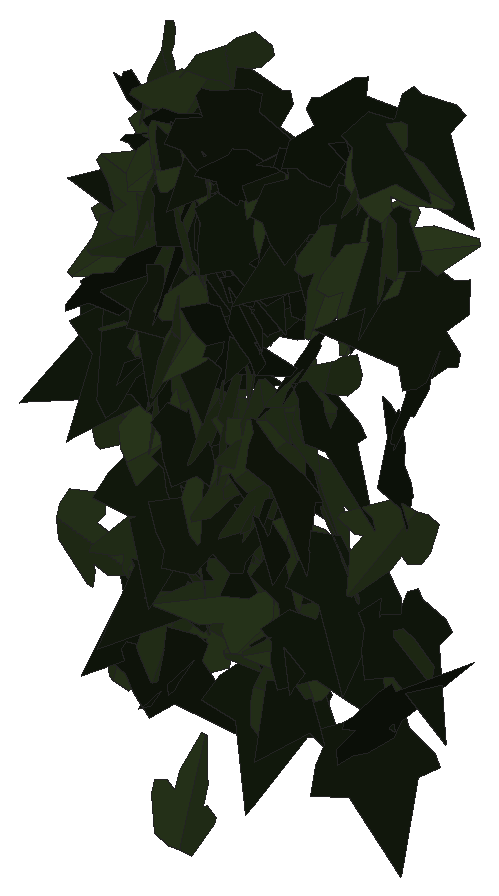
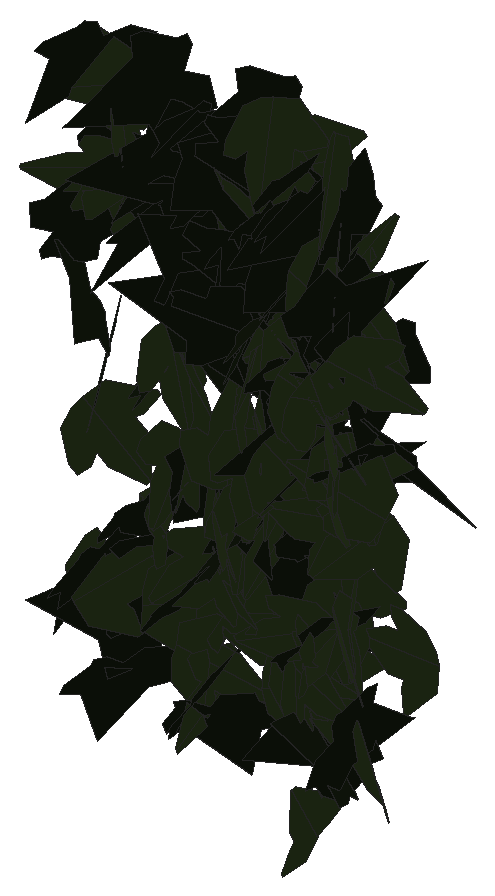
# SketchUp Ruby script. Lengths in inches.
U = 1.inch
M = Sketchup.active_model
def pt(a) = Geom::Point3d.new(a.map { |v| v * U })
def face(e, loops, mat)
  f = e.add_face(loops[0].map { |a| pt(a) })
  loops[1..].each { |l| e.add_face(l.map { |a| pt(a) }).erase! }
  f.material = f.back_material = mat if mat
  f
end
# faces: each face lists its corners as indices into pts; further lists are holes
def faces(e, pts, list, mat = nil) = list.each { |f| face(e, (f[0].is_a?(Array) ? f : [f]).map { |l| l.map { |i| pts[i] } }, mat) }
# xy, xz, yz: faces in a plane at the given z, y or x. An outline is a flat list of corners, or four numbers for a rectangle; further outlines are holes
def ring(l) = l.size == 4 ? [[l[0], l[1]], [l[2], l[1]], [l[2], l[3]], [l[0], l[3]]] : l.each_slice(2).to_a
def flat(e, list, mat, &to3) = list.each { |f| face(e, (f[0].is_a?(Array) ? f : [f]).map { |l| ring(l).map { |u, v| to3.(u, v) } }, mat) }
def xy(e, z, list, mat = nil) = flat(e, list, mat) { |x, y| [x, y, z] }
def xz(e, y, list, mat = nil) = flat(e, list, mat) { |x, z| [x, y, z] }
def yz(e, x, list, mat = nil) = flat(e, list, mat) { |y, z| [x, y, z] }
def lines(e, pts, list) = list.each { |a, b| e.add_line(pt(pts[a]), pt(pts[b])) }
# prism: a flat outline (further loops are holes) pulled along v
def prism(e, loops, v, mat = nil)
  f = face(e, loops, mat); d = Geom::Vector3d.new(v.map { |x| x * U })
  f.pushpull(f.normal.samedirection?(d) ? d.length : -d.length)
end
def box(e, o, s, mat = nil) = prism(e, [[o, [o[0] + s[0], o[1], o[2]], [o[0] + s[0], o[1] + s[1], o[2]], [o[0], o[1] + s[1], o[2]]]], [0, 0, s[2]], mat)
def at(x, y, z, deg = 0) = Geom::Transformation.translation(pt([x, y, z])) * Geom::Transformation.rotation(ORIGIN, Z_AXIS, deg.degrees)
def axes(o, x, y, z) = Geom::Transformation.new([*x, 0, *y, 0, *z, 0, *pt(o).to_a, 1])
def part(name) = M.definitions.add(name)
# library, detail: a bought-in or finely detailed component or shape, given as its bounding box
def library(name, o, s) = part(name).tap { |d| box(d.entities, o, s) }
def detail(e, o, s) = box(e.add_group.entities, o, s)
def put(e, d, t, mat = nil) = e.add_instance(d, t).tap { |i| i.material = mat if mat }
def group(e, t, mat = nil) = e.add_group.tap { |g| g.transformation = t; g.material = mat if mat }.entities
root = M.entities
M.materials.add("efeu1").color = [18, 25, 13]
M.materials.add("efeu2").color = [43, 57, 29]
c1 = part("ivyleaf_9")
p = [[1.54,2.16,1.25],[1.36,2.04,1.19],[-0.21,0.99,0.68],[-0.71,1.11,0.82],[-0.85,0.86,0.67],[-0.8,0.17,0.21],
  [-0.9,-0.01,0.1],[-0.67,-0.16,-0.02],[-0.08,-0.08,-0.05],[-0.03,-0.6,-0.4],[0.65,-0.88,-0.66],[0.83,-0.6,-0.49],
  [1.29,-0.42,-0.43],[1.8125,-0.07,-0.26],[1.21,0.44,0.15]]
faces(c1.entities,p,[[0,1,2,3,4,5,6,7,8,9,10,11,12,13,14]],"efeu1")
c2 = part("ivyleaf_10")
p = [[0,0.5,-0.03],[-0.0625,2.02,-0.43],[-0.19,2.01,-0.46],[-0.54,1.05,-0.29],[-0.52,0.625,-0.18],[-0.83,0.76,-0.28],
  [-1.16,0.64,-0.33],[-1.15,0.33,-0.24],[-0.77,-0.39,0.02],[-0.3,-0.51,0.16],[0.04,-0.48,0.23],[-0.02,2.01,-0.4375],
  [-0.06,2.01,-0.43],[0.04,-0.49,0.23],[0.67,-0.49,0.14],[1.38,0.36,-0.2],[1.375,0.51,-0.24],[0.81,0.65,-0.19],
  [0.62,0.59,-0.15],[0.6,1.09,-0.28],[0.5,1.23,-0.31]]
faces(c2.entities,p,[[0,1,2,3,4,5,6,7,8,9,10],[11,12,0,13,14,15,16,17,18,19,20]],"efeu2")
put(root,c1,axes([26,222.56,219.11],[-0.4769,0.10257,0.10975],[-0.10783,0.0206,-0.4878],[-0.10459,-0.48893,0.00247]))
put(root,c1,axes([27.44,222.25,222.61],[0.04677,0.071,-0.49272],[0.25531,0.42142,0.08496],[0.42735,-0.25954,0.00317]))
put(root,c2,axes([26.96,222.25,219.75],[0.05277,-0.33846,-0.36422],[-0.01811,0.36472,-0.34154],[0.49688,0.04924,0.02623]))
put(root,c1,axes([26.62,222.67,217.6875],[-0.32572,-0.33531,-0.17742],[0.13158,0.11946,-0.46735],[0.3558,-0.35114,0.01042]))
put(root,c2,axes([27.1,222.21,213.6875],[0.02192,0.38608,-0.31696],[0.03124,0.31558,0.38657],[0.49854,-0.03675,-0.01029]))
put(root,c1,axes([26.18,222.25,220.25],[0.13268,0.48116,-0.02974],[-0.0089,-0.02839,-0.49911],[-0.48199,0.13298,0.00103]))
put(root,c2,axes([29.8,222.7,218.16],[-0.20695,-0.34897,0.29222],[-0.12821,-0.26331,-0.40525],[0.43673,-0.24267,0.01951]))
put(root,c1,axes([29.0625,222.75,217.375],[-0.04611,-0.49762,0.01589],[0.00134,-0.01609,-0.49974],[0.49787,-0.04604,0.00282]))
put(root,c2,axes([28.99,222.66,221.34],[0.18709,0.39205,-0.24758],[-0.08922,-0.23154,-0.43408],[-0.45501,0.20661,-0.01668]))
put(root,c2,axes([26.875,222.55,222],[0.38106,-0.00662,-0.32365],[-0.32328,0.01813,-0.381],[0.01678,0.49963,0.00953]))
put(root,c1,axes([27.43,222.35,217.21],[-0.46658,0.06612,0.16711],[0.16511,-0.02591,0.47124],[0.07098,0.49493,0.00234]))
put(root,c2,axes([25.32,222.61,216.62],[-0.07292,0.04696,-0.49242],[0.44472,-0.2117,-0.08605],[-0.21657,-0.45053,-0.0109]))
put(root,c2,axes([26.47,222.54,217.01],[-0.29156,-0.40555,0.02281],[-0.0134,-0.01846,-0.49948],[0.40597,-0.29187,-0.00011]))
put(root,c2,axes([26.36,222.53,220.75],[-0.27482,-0.05765,0.4137],[-0.40528,-0.08308,-0.2808],[0.10112,-0.48967,-0.00107]))
put(root,c2,axes([27.125,222.7,219.99],[0.26993,0.30188,-0.29327],[-0.18987,-0.22359,-0.40492],[-0.37562,0.32996,-0.00608]))
put(root,c1,axes([28.76,222.65,219.31],[0.2713,-0.41997,0.00461],[0.0025,-0.00387,-0.49998],[0.41999,0.27131,0]))
put(root,c2,axes([27.6,222.75,216.51],[0.03345,0.0607,-0.49517],[-0.44165,-0.22719,-0.05768],[-0.232,0.44125,0.03841]))
put(root,c2,axes([26.92,222.71,222.54],[-0.23985,-0.37338,0.23035],[-0.09067,-0.21468,-0.44237],[0.42925,-0.25398,0.03527]))
put(root,c2,axes([29.45,222.63,221.3],[0.31072,0.35782,-0.15943],[-0.10236,-0.12227,-0.47389],[-0.37812,0.32714,-0.00273]))
put(root,c1,axes([26.65,222.93,216.49],[-0.2778,-0.34146,0.23713],[-0.12438,-0.20387,-0.43928],[0.39668,-0.30305,0.02833]))
put(root,c1,axes([27.11,222.59,216.83],[-0.15132,0.06294,0.47238],[0.38889,-0.27015,0.16057],[0.27544,0.416,0.03281]))
put(root,c2,axes([26.68,222.66,216.0625],[-0.23025,-0.42995,0.11013],[-0.04507,-0.10078,-0.48766],[0.44154,-0.23449,0.00765]))
put(root,c2,axes([28.72,222.86,216.29],[0.01115,0.03174,-0.49887],[-0.3673,-0.33794,-0.02971],[-0.33906,0.36713,0.01578]))
put(root,c2,axes([26.32,222.76,221],[-0.01761,0.38951,0.313],[-0.01688,-0.31348,0.38916],[0.4994,0.00314,0.02419]))
put(root,c2,axes([29.5,222.67,221.69],[0.43821,-0.2295,0.07282],[0.06865,-0.02585,-0.49459],[0.23078,0.44347,0.00885]))
put(root,c2,axes([27.96,222.73,218.4375],[-0.27935,-0.2078,0.35886],[-0.28085,-0.22354,-0.34807],[0.3051,-0.39604,0.00816]))
put(root,c1,axes([28.07,222.83,218.39],[0.14621,-0.46138,0.1255],[0.04153,-0.11848,-0.48398],[0.47634,0.15195,0.00368]))
put(root,c2,axes([26.51,222.4375,221.4375],[0.1581,-0.38696,-0.27435],[-0.02032,0.2834,-0.41143],[0.47391,0.14124,0.07388]))
put(root,c2,axes([26.97,222.74,221.39],[-0.26885,0.32414,-0.26954],[0.09475,-0.26505,-0.41324],[-0.41078,-0.27328,0.08109]))
put(root,c2,axes([26.95,222.45,221.16],[-0.23786,0.42093,0.12743],[-0.07019,0.10669,-0.48342],[-0.43416,-0.24786,0.00834]))
put(root,c1,axes([29.39,222.76,221.79],[-0.39357,-0.18904,-0.24365],[0.21736,0.11019,-0.43659],[0.21877,-0.44958,-0.00455]))
put(root,c2,axes([27.35,222.8125,218.93],[0.24503,-0.3728,0.22579],[0.15753,-0.16577,-0.44464],[0.40638,0.28904,0.03622]))
put(root,c1,axes([28.76,222.95,221.39],[-0.40449,-0.22677,0.18698],[-0.14051,-0.13019,-0.46185],[0.25816,-0.42617,0.04159]))
put(root,c1,axes([27,222.53,219.64],[0.19931,0.13211,-0.43911],[0.35027,0.26515,0.23876],[0.29595,-0.40279,0.01314]))
put(root,c1,axes([28.77,222.53,216.64],[-0.11176,-0.1846,-0.45104],[0.19886,0.40519,-0.21511],[0.44493,-0.22747,-0.01715]))
put(root,c1,axes([27.5625,222.65,221.32],[0.12738,-0.42197,-0.23605],[-0.07208,0.2248,-0.44076],[0.4781,0.14632,-0.00355]))
put(root,c1,axes([26.03,223,218.98],[-0.31516,-0.35453,0.15808],[-0.05816,-0.15819,-0.47074],[0.38379,-0.3151,0.05847]))
put(root,c1,axes([26.12,222.86,221.87],[0.11032,-0.18095,0.45287],[0.30189,-0.33931,-0.20912],[0.38301,0.31957,0.03439]))
put(root,c1,axes([29.53,223.04,218.68],[0.00274,-0.12171,0.48495],[0.00376,-0.48494,-0.12173],[0.49998,0.00431,-0.00174]))
put(root,c1,axes([27.5,222.7,220.27],[0.02691,0.08722,-0.4916],[-0.41095,-0.27572,-0.07142],[-0.28355,0.40788,0.05685]))
put(root,c1,axes([26.8,222.86,219.98],[-0.09443,-0.4744,-0.12661],[0.04396,0.12024,-0.48333],[0.48903,-0.10241,0.019]))
put(root,c2,axes([28.22,222.88,218.96],[0.15788,-0.1327,-0.45548],[0.35079,-0.29053,0.20624],[-0.3194,-0.38468,0.00136]))
put(root,c1,axes([26.4375,222.59,215.45],[-0.01835,0.00795,-0.4996],[0.37844,0.32666,-0.0087],[0.32626,-0.37846,-0.018]))
put(root,c1,axes([27.92,222.62,222.07],[0.12586,0.38928,-0.28743],[-0.14729,-0.25209,-0.40591],[-0.46094,0.18685,0.05121]))
put(root,c2,axes([27.91,222.77,221.68],[0.47232,-0.10327,0.12748],[0.12571,-0.02185,-0.48345],[0.10542,0.48873,0.00533]))
put(root,c1,axes([30.08,223.02,220.5625],[-0.17501,-0.10931,0.45544],[-0.39945,-0.21903,-0.20606],[0.24456,-0.43598,-0.01067]))
put(root,c2,axes([26.01,222.94,216.89],[0.11765,-0.18679,0.44863],[0.39525,-0.23177,-0.20015],[0.28273,0.40174,0.09312]))
put(root,c1,axes([28.49,222.42,222.13],[0.13182,-0.1253,-0.46575],[-0.1193,0.45936,-0.15735],[0.46732,0.15261,0.09121]))
put(root,c1,axes([28.625,222.6875,220.02],[-0.33159,0.35975,-0.10309],[0.06936,-0.07628,-0.48926],[-0.36774,-0.33877,0.00068]))
put(root,c1,axes([29.52,222.33,215.7],[-0.01124,0.40602,-0.29158],[-0.02728,0.29072,0.40588],[0.49913,0.02503,0.01561]))
put(root,c2,axes([27.9,222.71,217.9],[-0.02474,-0.49457,-0.06923],[-0.00166,0.0694,-0.49516],[0.49938,-0.02427,-0.00508]))
put(root,c1,axes([26.67,223.01,220.95],[-0.14971,0.01589,-0.4768],[0.39157,-0.28136,-0.13233],[-0.27251,-0.41302,0.0718]))
put(root,c1,axes([29.33,222.81,215.22],[-0.07473,-0.4392,-0.22697],[0.05369,0.22099,-0.44529],[0.49146,-0.09093,0.01413]))
put(root,c1,axes([26.47,222.98,219.99],[-0.19759,-0.45845,-0.02799],[0.01603,0.02357,-0.49919],[0.45902,-0.19817,0.00539]))
put(root,c2,axes([26.63,222.93,216.2],[-0.31493,0.02047,0.38782],[0.3555,-0.18581,0.29849],[0.15634,0.46374,0.10248]))
put(root,c1,axes([26.84,222.71,218.47],[0.24473,-0.36784,-0.23409],[-0.06623,0.23396,-0.43689],[0.43095,0.24485,0.06579]))
put(root,c1,axes([27.85,222.91,222.37],[-0.13415,-0.13181,-0.46328],[-0.34271,-0.31181,0.18795],[-0.33846,0.36797,-0.00669]))
put(root,c2,axes([28.63,222.83,219.55],[-0.14413,-0.47674,0.04413],[-0.01393,-0.04189,-0.49805],[0.47857,-0.1448,-0.0012]))
put(root,c1,axes([26.7,222.84,221.16],[0.20396,-0.44159,-0.11574],[-0.0289,0.11402,-0.48597],[0.45559,0.20493,0.02099]))
put(root,c2,axes([26.74,222.71,218.65],[0.32117,-0.07394,-0.37601],[-0.33875,0.1746,-0.32368],[0.17917,0.46265,0.06205]))
put(root,c1,axes([27.71,222.8,219.79],[0.02854,-0.41131,0.28286],[-0.01569,0.28244,0.41229],[-0.49894,-0.0324,0.00322]))
put(root,c2,axes([26.13,223.09,218.59],[0.13768,-0.13782,0.46049],[0.32118,-0.33,-0.19479],[0.35762,0.34943,-0.00234]))
put(root,c2,axes([27.77,222.96,218.36],[-0.21033,-0.43069,-0.14236],[-0.05878,-0.12971,0.47929],[-0.44978,0.21835,0.00393]))
put(root,c2,axes([26.22,222.86,220.39],[0.43895,-0.23751,-0.03021],[-0.02731,0.013,-0.49908],[0.23786,0.4398,-0.00156]))
put(root,c1,axes([27.61,223.13,217.48],[0.05224,-0.36236,0.34054],[0.11448,-0.32445,-0.36281],[0.48391,0.11588,0.04907]))
put(root,c2,axes([26.13,223.125,218.92],[-0.10642,0.08328,-0.48139],[0.13192,-0.46948,-0.11038],[-0.4704,-0.1505,0.07796]))
put(root,c1,axes([26.52,222.52,222],[0.41851,0.2001,0.18658],[0.16371,0.09005,-0.46378],[-0.21921,0.44928,0.00986]))
put(root,c1,axes([28.02,223.22,215.39],[-0.07979,-0.36859,0.32829],[-0.03649,-0.32723,-0.37628],[0.49224,-0.08401,0.02532]))
put(root,c2,axes([26.73,222.91,220.35],[-0.40274,-0.21352,0.20545],[-0.15083,-0.15068,-0.45227],[0.25506,-0.42626,0.05696]))
put(root,c2,axes([26.09,222.87,219.02],[-0.41351,-0.22532,0.16804],[-0.14059,-0.09303,-0.47072],[0.24339,-0.43655,0.01358]))
put(root,c2,axes([28.56,223.05,217.36],[-0.02483,-0.12702,0.48296],[0.45452,-0.20605,-0.03082],[0.20686,0.4375,0.1257]))
put(root,c2,axes([29.35,222.71,222.54],[0.12436,0.05107,0.48159],[0.42425,0.22829,-0.13377],[-0.23354,0.4419,0.01345]))
put(root,c1,axes([27.08,223.24,221.93],[-0.13626,-0.3665,0.31162],[-0.11463,-0.28982,-0.39098],[0.46722,-0.17799,-0.00505]))
put(root,c2,axes([27.55,222.8,217.89],[-0.20717,-0.44073,-0.11329],[0.06183,0.09606,-0.48677],[0.45084,-0.2157,0.0147]))
put(root,c2,axes([26.34,222.57,217.97],[0.13136,0.09878,-0.47221],[0.3507,0.31653,0.16377],[0.33129,-0.37424,0.01387]))
put(root,c2,axes([25.8,222.81,218.18],[-0.36868,-0.04988,-0.33404],[0.33477,0.01155,-0.37121],[0.04475,-0.49737,0.02488]))
put(root,c1,axes([28.2,223.2,216.7],[-0.0675,-0.46849,0.16112],[0.01403,-0.16435,-0.47201],[0.49522,-0.0592,0.03533]))
put(root,c1,axes([26.98,222.78,218.14],[-0.03875,-0.1482,-0.47596],[0.29233,0.37994,-0.1421],[0.40379,-0.28928,0.0572]))
put(root,c1,axes([27.85,223.08,215.31],[-0.32872,-0.36118,-0.10719],[0.07312,0.07838,-0.48837],[0.36959,-0.33675,0.00129]))
put(root,c2,axes([26.4,223.23,219.76],[-0.15733,-0.19687,0.43184],[0.07325,-0.45957,-0.18283],[0.46891,0.00573,0.17345]))
put(root,c2,axes([27.03,222.86,215.77],[-0.08152,0.02095,-0.49286],[-0.48336,0.09642,0.08405],[0.09857,0.49017,0.00454]))
put(root,c1,axes([25.94,223.29,215.66],[0.04852,-0.15577,-0.47263],[0.24104,-0.4081,0.15924],[-0.43537,-0.2433,0.03549]))
put(root,c2,axes([27.14,222.67,217.77],[0.043,0.44155,0.23062],[0.02922,0.22885,-0.44359],[-0.49729,0.05162,-0.00612]))
put(root,c1,axes([27.3125,222.69,219.84],[-0.10432,0.21625,0.43858],[-0.31603,0.31239,-0.2292],[-0.37315,-0.32503,0.07151]))
put(root,c2,axes([28.2,222.99,215.8],[-0.07647,-0.04126,0.49239],[-0.4612,-0.17285,-0.0861],[0.17733,-0.46736,-0.01162]))
put(root,c2,axes([27.74,223.01,217.76],[0.16517,-0.47027,0.03956],[0.01245,-0.03756,-0.49843],[0.47177,0.16563,-0.00069]))
put(root,c1,axes([27.98,222.89,218.33],[0.13982,0.19676,-0.43788],[-0.35013,-0.27022,-0.23322],[-0.32842,0.37185,0.06221]))
put(root,c1,axes([26.45,222.62,219.15],[0.07975,0.07671,-0.4876],[0.0979,0.48165,0.09179],[0.48379,-0.11012,0.0618]))
put(root,c2,axes([29.61,223,216.17],[-0.31741,0.03069,-0.38511],[-0.38624,-0.01474,0.31717],[0.00811,0.49884,0.03307]))
put(root,c2,axes([26.73,222.93,220.3],[0.2562,-0.02016,0.4289],[0.42535,0.08012,-0.25032],[-0.05863,0.49313,0.05821]))
put(root,c2,axes([26.84,223.21,218.88],[-0.1798,-0.34659,0.31232],[-0.02752,-0.32625,-0.37789],[0.46574,-0.15308,0.09824]))
put(root,c1,axes([29.61,222.85,223.05],[0.04237,-0.3143,-0.38655],[0.05151,0.38863,-0.31035],[0.49553,-0.01353,0.06531]))
put(root,c2,axes([28.13,222.85,216.59],[0.02825,-0.00522,0.49917],[-0.4951,0.06364,0.02868],[-0.06383,-0.49591,-0.00157]))
put(root,c1,axes([27.02,223.17,220.67],[0.17758,-0.45409,0.11078],[0.06136,-0.09483,-0.48708],[0.46336,0.18658,0.02205]))
put(root,c1,axes([27.82,223.18,220.52],[-0.41629,-0.26918,-0.06516],[0.05705,0.03178,-0.49572],[0.27102,-0.42016,0.00426]))
put(root,c1,axes([26.24,223.28,220.73],[-0.08505,-0.03583,0.49141],[-0.39623,-0.29143,-0.08982],[0.29286,-0.40471,0.02117]))
put(root,c1,axes([28.26,222.68,220.61],[-0.08467,-0.09844,0.48284],[0.34054,0.34242,0.12953],[-0.35618,0.35079,0.00906]))
put(root,c2,axes([27.15,222.79,218.71],[0.04662,-0.40121,-0.29471],[-0.02637,0.2936,-0.40386],[0.49712,0.0532,0.00621]))
put(root,c2,axes([26.57,223.3,219.95],[-0.06499,-0.32917,0.3707],[0.11291,-0.37388,-0.3122],[0.48273,0.04313,0.12294]))
put(root,c2,axes([27.375,222.93,218.64],[-0.48974,-0.0971,0.02697],[-0.02643,-0.0054,-0.49927],[0.09725,-0.49045,0.00015]))
put(root,c2,axes([26.88,222.96,216.12],[-0.12242,0.01452,0.48457],[-0.48248,-0.05234,-0.12032],[0.04723,-0.49704,0.02682]))
put(root,c2,axes([26.46,223.28,221.3],[0.04818,-0.34094,0.36254],[0.18366,-0.32635,-0.33131],[0.46254,0.16509,0.09379]))
put(root,c2,axes([26.52,222.95,216.69],[-0.16873,-0.08882,-0.46221],[0.47035,-0.01364,-0.16908],[0.01743,-0.49186,0.08816]))
put(root,c1,axes([28.72,222.6,222.82],[0.04009,0.16184,-0.47138],[-0.04347,0.47224,0.15844],[0.49649,0.02828,0.05193]))
put(root,c2,axes([25.71,222.93,214.98],[0.44143,-0.22897,0.05214],[-0.03709,0.04164,0.49688],[-0.23188,-0.44254,0.01978]))
put(root,c1,axes([26.63,222.98,222.17],[0.1845,-0.41099,-0.2169],[-0.06871,0.20668,-0.45007],[0.45961,0.19588,0.01979]))
put(root,c2,axes([29.1875,222.98,222.36],[0.12659,-0.47499,-0.09141],[-0.01467,0.09068,-0.49149],[0.48349,0.12711,0.00902]))
put(root,c1,axes([27.77,222.77,220.17],[0.15515,0.02352,0.47474],[0.46386,0.1015,-0.15663],[-0.10374,0.48902,0.00967]))
put(root,c2,axes([25.9,223.16,220.33],[0.268,0.1402,-0.39815],[-0.35706,-0.17624,-0.3024],[-0.22513,0.44641,0.00566]))
put(root,c2,axes([28.01,222.64,215.47],[0.01757,0.25505,0.4297],[-0.09648,0.4236,-0.24749],[-0.49029,-0.07422,0.0641]))
put(root,c2,axes([28.46,222.96,218.25],[-0.45761,0.18112,-0.08825],[0.07717,-0.04473,-0.49198],[-0.18611,-0.46389,0.01298]))
put(root,c2,axes([26.32,222.84,222.71],[0.12474,-0.40128,-0.27095],[0.0043,0.2807,-0.41375],[0.48417,0.10089,0.07348]))
put(root,c1,axes([26.73,222.79,219.47],[-0.24442,0.2947,0.32157],[-0.19681,0.25445,-0.38278],[-0.38926,-0.31369,-0.00839]))
put(root,c2,axes([27.26,223.31,219.375],[0.02258,-0.13073,0.48208],[0.35494,-0.33533,-0.10756],[0.35144,0.34707,0.07766]))
put(root,c1,axes([29.96,222.64,219.67],[-0.01183,0.25628,0.42916],[-0.07007,0.42419,-0.25525],[-0.49492,-0.06618,0.02588]))
put(root,c2,axes([29.49,222.79,221.43],[0.08741,-0.07333,-0.48681],[0.42937,0.25323,0.03896],[0.24083,-0.42485,0.10724]))
put(root,c2,axes([25.98,223.14,217.03],[0.26497,-0.41882,0.06622],[0.04041,-0.05278,-0.49556],[0.42209,0.26797,0.00588]))
put(root,c1,axes([29.49,223.06,216.72],[0.15516,-0.43256,-0.19702],[-0.07096,0.18384,-0.45953],[0.46999,0.17056,-0.00434]))
put(root,c2,axes([27.12,222.98,222.94],[-0.22931,-0.43134,-0.10661],[0.04801,0.09521,-0.4885],[0.44171,-0.23427,-0.00224]))
put(root,c2,axes([25.8,222.94,218.52],[-0.15877,-0.10687,0.46192],[0.41599,0.20231,0.18979],[-0.22747,0.44458,0.02467]))
put(root,c1,axes([27.87,223.18,221.12],[-0.41847,0.00334,0.27362],[-0.27361,0.0029,-0.41849],[-0.00439,-0.49998,-0.0006]))
put(root,c2,axes([27.86,222.98,217.125],[-0.34206,-0.02313,-0.36395],[0.36404,0.00815,-0.34265],[0.02179,-0.4994,0.01127]))
put(root,c1,axes([26.53,222.72,215.1],[-0.30661,0.38013,-0.10721],[-0.06735,0.08341,0.48837],[0.38917,0.31392,0.00006]))
put(root,c1,axes([26.65,223,221.41],[0.15492,0.32743,-0.34466],[-0.21255,-0.27654,-0.35826],[-0.42523,0.25752,0.05351]))
put(root,c1,axes([28.625,222.98,221.28],[0.1759,-0.36676,-0.29077],[-0.02286,0.30352,-0.39668],[0.46748,0.15284,0.09001]))
put(root,c1,axes([28.29,222.8125,221.92],[0.33603,0.08306,0.36081],[0.35049,0.08566,-0.34615],[-0.11932,0.48555,-0.00066]))
